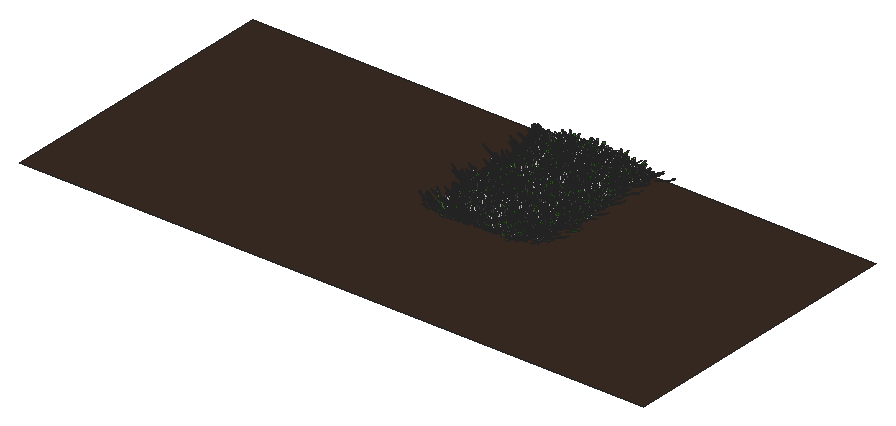
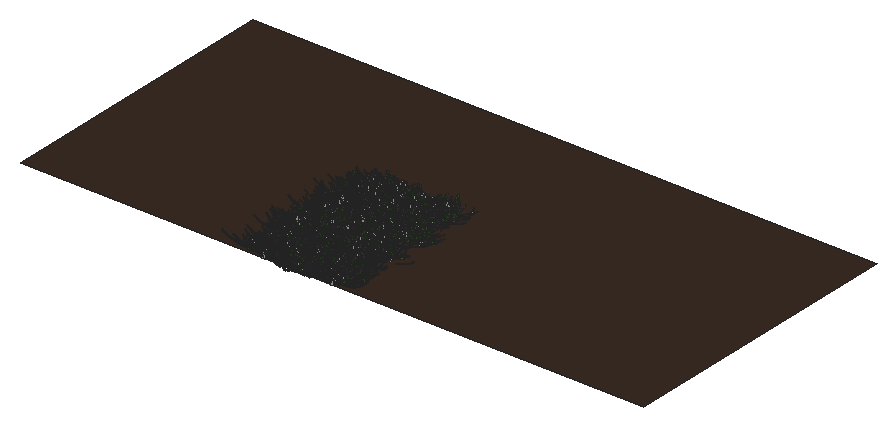
# SketchUp Ruby script. Lengths in inches.
U = 1.inch
M = Sketchup.active_model
def pt(a) = Geom::Point3d.new(a.map { |v| v * U })
def face(e, loops, mat)
  f = e.add_face(loops[0].map { |a| pt(a) })
  loops[1..].each { |l| e.add_face(l.map { |a| pt(a) }).erase! }
  f.material = f.back_material = mat if mat
  f
end
# faces: each face lists its corners as indices into pts; further lists are holes
def faces(e, pts, list, mat = nil) = list.each { |f| face(e, (f[0].is_a?(Array) ? f : [f]).map { |l| l.map { |i| pts[i] } }, mat) }
# xy, xz, yz: faces in a plane at the given z, y or x. An outline is a flat list of corners, or four numbers for a rectangle; further outlines are holes
def ring(l) = l.size == 4 ? [[l[0], l[1]], [l[2], l[1]], [l[2], l[3]], [l[0], l[3]]] : l.each_slice(2).to_a
def flat(e, list, mat, &to3) = list.each { |f| face(e, (f[0].is_a?(Array) ? f : [f]).map { |l| ring(l).map { |u, v| to3.(u, v) } }, mat) }
def xy(e, z, list, mat = nil) = flat(e, list, mat) { |x, y| [x, y, z] }
def xz(e, y, list, mat = nil) = flat(e, list, mat) { |x, z| [x, y, z] }
def yz(e, x, list, mat = nil) = flat(e, list, mat) { |y, z| [x, y, z] }
def lines(e, pts, list) = list.each { |a, b| e.add_line(pt(pts[a]), pt(pts[b])) }
# prism: a flat outline (further loops are holes) pulled along v
def prism(e, loops, v, mat = nil)
  f = face(e, loops, mat); d = Geom::Vector3d.new(v.map { |x| x * U })
  f.pushpull(f.normal.samedirection?(d) ? d.length : -d.length)
end
def box(e, o, s, mat = nil) = prism(e, [[o, [o[0] + s[0], o[1], o[2]], [o[0] + s[0], o[1] + s[1], o[2]], [o[0], o[1] + s[1], o[2]]]], [0, 0, s[2]], mat)
def at(x, y, z, deg = 0) = Geom::Transformation.translation(pt([x, y, z])) * Geom::Transformation.rotation(ORIGIN, Z_AXIS, deg.degrees)
def axes(o, x, y, z) = Geom::Transformation.new([*x, 0, *y, 0, *z, 0, *pt(o).to_a, 1])
def part(name) = M.definitions.add(name)
# library, detail: a bought-in or finely detailed component or shape, given as its bounding box
def library(name, o, s) = part(name).tap { |d| box(d.entities, o, s) }
def detail(e, o, s) = box(e.add_group.entities, o, s)
def put(e, d, t, mat = nil) = e.add_instance(d, t).tap { |i| i.material = mat if mat }
def group(e, t, mat = nil) = e.add_group.tap { |g| g.transformation = t; g.material = mat if mat }.entities
root = M.entities
M.materials.add("Material82").color = [68, 110, 58]
M.materials.add("Material83").color = [48, 90, 38]
M.materials.add("Material84").color = [68, 110, 48]
M.materials.add("Material85").color = [48, 90, 48]
M.materials.add("Material86").color = [58, 110, 58]
M.materials.add("Material87").color = [58, 90, 38]
M.materials.add("Material88").color = [68, 100, 58]
M.materials.add("Material89").color = [48, 100, 38]
M.materials.add("top-soil").color = [58, 44, 36]
c1 = part("grass00")
p = [[-0.6875,0.15,0],[-0.56,0.08,5.52],[-0.04,0.03,2.76],[0.48,-0.02,0],[0.35,-0.02,5.52],[-0.1,-0.14,5.52],
  [-0.12,0.65,8.37],[-0.42,0.65,8.37]]
faces(c1.entities,p,[[0,1,2,3],[3,2,4],[1,5,2],[5,4,2],[1,6,5],[4,5,6],[7,6,1]])
c2 = part("Group16\#1")
put(c2.entities,c1,axes([1.44,-0.61,-0.01],[0.05352,0.12609,0],[-0.10704,0.04543,0.07239],[0.06664,-0.02828,0.11628]),"Material85")
put(c2.entities,c1,axes([0.76,-0.15,-0.01],[0.04676,0.24062,0],[-0.23162,0.04501,0.06642],[0.0652,-0.01267,0.23595]),"Material82")
put(c2.entities,c1,axes([0.79,0.01,-0.01],[-0.00606,0.34651,0],[-0.34381,-0.00602,0.0432],[0.04319,0.00076,0.34386]))
put(c2.entities,c1,axes([1,0.23,-0.01],[-0.07192,0.31144,0],[-0.28722,-0.06632,0.1236],[0.12043,0.02781,0.29478]),"Material84")
put(c2.entities,c1,axes([1.66,0.77,-0.01],[-0.13828,0.29651,0],[-0.21551,-0.1005,0.22471],[0.20365,0.09498,0.23779]),"Material89")
put(c2.entities,c1,axes([0.6875,0.52,-0.01],[-0.18126,0.24051,0],[-0.22746,-0.17142,0.09788],[0.07817,0.05891,0.28481]),"Material84")
put(c2.entities,c1,axes([0.68,0.78,-0.01],[-0.215,0.18688,0],[-0.12385,-0.14248,0.21334],[0.13995,0.16101,0.18878]),"Material82")
put(c2.entities,c1,axes([0.56,1,-0.01],[-0.13756,0.07624,0],[-0.06159,-0.11112,0.0927],[0.04494,0.08108,0.12705]),"Material84")
put(c2.entities,c1,axes([0.2,0.64,-0.01],[-0.23729,0.07254,0],[-0.05711,-0.18681,0.153],[0.04473,0.14632,0.19535]),"Material89")
put(c2.entities,c1,axes([0.0625,0.72,-0.01],[-0.28874,0.02525,0],[-0.02179,-0.24916,0.14647],[0.01276,0.14591,0.25012]),"Material82")
put(c2.entities,c1,axes([-0.08,0.62,-0.01],[-0.34089,-0.04187,0],[0.03255,-0.26504,0.216],[-0.02633,0.21439,0.26703]),"Material89")
put(c2.entities,c1,axes([-0.34,0.98,-0.01],[-0.14314,-0.0493,0],[0.04397,-0.12769,0.06843],[-0.02228,0.0647,0.13505]),"Material89")
put(c2.entities,c1,axes([-0.87,1.45,-0.01],[-0.23488,-0.14114,0],[0.13761,-0.22901,0.06087],[-0.03135,0.05217,0.26717]))
put(c2.entities,c1,axes([-0.72,0.77,-0.01],[-0.14208,-0.13251,0],[0.07209,-0.0773,0.16301],[-0.11118,0.11922,0.1057]),"Material89")
put(c2.entities,c1,axes([-0.62,0.43,-0.01],[-0.14845,-0.21203,0],[0.18654,-0.13061,0.12304],[-0.10079,0.07057,0.22772]),"Material82")
put(c2.entities,c1,axes([-0.68,0.29,-0.01],[-0.13639,-0.32136,0],[0.31723,-0.13464,0.05579],[-0.05136,0.0218,0.34462]),"Material83")
put(c2.entities,c1,axes([-0.64,0.125,-0.01],[-0.0458,-0.23569,0],[0.22124,-0.043,0.08276],[-0.08124,0.01579,0.22538]),"Material86")
put(c2.entities,c1,axes([-1.6,-0.03,-0.01],[0.00576,-0.32897,0],[0.27526,0.00482,0.18018],[-0.18015,-0.00315,0.2753]),"Material84")
put(c2.entities,c1,axes([-1.36,-0.31,-0.01],[0.05718,-0.24765,0],[0.18172,0.04196,0.17267],[-0.16825,-0.03885,0.1865]),"Material89")
put(c2.entities,c1,axes([-1.54,-0.72,-0.01],[0.06537,-0.14017,0],[0.13555,0.06321,0.03939],[-0.0357,-0.01665,0.14956]))
put(c2.entities,c1,axes([-1.19,-0.9,-0.01],[0.09597,-0.12735,0],[0.11214,0.08451,0.07557],[-0.06035,-0.04548,0.14042]),"Material88")
put(c2.entities,c1,axes([-0.47,-0.54,-0.01],[0.11588,-0.10072,0],[0.0618,0.0711,0.12124],[-0.07953,-0.0915,0.0942]))
put(c2.entities,c1,axes([-0.47,-0.84,-0.01],[0.11927,-0.0661,0],[0.06603,0.11913,0.00646],[-0.00313,-0.00565,0.13621]),"Material84")
put(c2.entities,c1,axes([-0.38,-1.24,-0.01],[0.28037,-0.08571,0],[0.0618,0.20215,0.20315],[-0.05939,-0.19428,0.21139]),"Material88")
put(c2.entities,c1,axes([-0.06,-0.66,-0.01],[0.22719,-0.01987,0],[0.01247,0.14255,0.17758],[-0.01547,-0.17691,0.1431]),"Material87")
put(c2.entities,c1,axes([0.11,-0.89,-0.01],[0.14882,0.01828,0],[-0.01058,0.08611,0.12229],[0.01491,-0.12138,0.08676]),"Material85")
put(c2.entities,c1,axes([0.25,-0.72,-0.01],[0.20481,0.07053,0],[-0.06206,0.18022,0.10291],[0.03351,-0.0973,0.1906]),"Material85")
put(c2.entities,c1,axes([0.85,-1.42,-0.01],[0.16481,0.09904,0],[-0.09472,0.15762,0.05616],[0.02893,-0.04814,0.18389]),"Material84")
put(c2.entities,c1,axes([1.01,-1.09,-0.01],[0.21858,0.20385,0],[-0.17495,0.1876,0.15339],[0.10462,-0.11218,0.25652]),"Material89")
put(c2.entities,c1,axes([1.01,-0.71,-0.01],[0.08733,0.12473,0],[-0.06445,0.04512,0.13037],[0.1068,-0.07477,0.07867]),"Material85")
c3 = part("Group15\#1")
put(c3.entities,c2,at(0,0,0))
c4 = part("3darcstudiotree_grass00\#1")
put(c4.entities,c3,at(0,0,0))
xy(root,-29.74,[[596.27,940.12,839.3,1053.55]],"top-soil")
put(root,c4,axes([716.37,1016.65,-29.74],[4.10776,0.45174,0],[-0.96091,1.35899,-0.03867],[-0.06802,0.0962,1.75619]))
put(root,c4,axes([716.7,1044.86,-29.74],[0.30119,1.56993,0],[-3.74927,0.11187,-0.04286],[-0.21599,0.00644,1.42447]))
put(root,c4,axes([718.33,1014.64,-29.74],[-3.02492,-1.16677,0],[2.80082,-1.12934,-0.0483],[0.17838,-0.07192,1.58573]))
put(root,c4,axes([717.53,1046.92,-29.74],[3.50639,-1.07574,0],[2.8139,1.42651,-0.05588],[0.16686,0.08459,1.67045]))
put(root,c4,axes([717.03,996.91,-29.74],[-0.3994,1.69229,0],[-4.36532,-0.16024,-0.02425],[-0.12976,-0.00476,1.76617]))
put(root,c4,axes([718.91,1050.84,-29.74],[-0.91614,-1.55858,0],[4.47177,-0.40881,-0.01344],[0.0544,-0.00497,1.42931]))
put(root,c4,axes([718.23,1031.09,-29.74],[-3.80907,0.85988,0],[-1.7501,-1.20575,-0.03218],[-0.10036,-0.06914,1.65786]))
put(root,c4,axes([718.77,1001.97,-29.74],[1.67083,-1.60234,0],[3.7829,0.6135,-0.00107],[0.00454,0.00074,1.41133]))
put(root,c4,axes([718.07,1049.21,-29.74],[-1.98309,1.36521,0],[-3.29696,-0.74485,-0.00674],[-0.03007,-0.00679,1.46389]))
put(root,c4,axes([718.36,1011.9,-29.74],[-1.6341,1.38385,0],[-3.29524,-0.60518,-0.01596],[-0.09907,-0.01819,1.86544]))
put(root,c4,axes([718.59,1017.96,-29.74],[-1.88391,1.25543,0],[-3.77395,-0.8808,-0.04665],[-0.1806,-0.04215,1.47851]))
put(root,c4,axes([719.67,1041.09,-29.74],[-3.20908,-0.65771,0],[1.52004,-1.1535,-0.02241],[0.0705,-0.0535,1.68548]))
put(root,c4,axes([718.79,1030.31,-29.74],[2.49471,1.02577,0],[-2.71621,1.02741,-0.02632],[-0.13149,0.04974,1.95302]))
put(root,c4,axes([719.14,1037.94,-29.74],[4.09109,-0.59758,0],[1.20224,1.2801,-0.03178],[0.07676,0.08173,1.80429]))
put(root,c4,axes([718.95,1005.53,-29.74],[2.32026,0.93484,0],[-2.86948,1.10768,-0.01876],[-0.07886,0.03044,1.77063]))
put(root,c4,axes([719.68,1024.48,-29.74],[0.18236,1.53314,0],[-4.12116,0.07624,-0.04808],[-0.2649,0.0049,1.70557]))
put(root,c4,axes([719.14,1028.03,-29.74],[1.69594,1.55136,0],[-4.25972,0.72425,-0.01792],[-0.06344,0.01079,1.34035]))
put(root,c4,axes([721.83,1040.77,-29.74],[-0.92548,-1.44714,0],[3.73119,-0.37112,-0.02503],[0.12441,-0.01237,1.47852]))
put(root,c4,axes([721.37,1011.59,-29.74],[-3.65717,1.04753,0],[-2.10189,-1.14131,-0.02785],[-0.11272,-0.06121,1.84622]))
put(root,c4,axes([721.35,1023.08,-29.74],[2.69686,-1.18339,0],[2.47302,0.87653,-0.01288],[0.05957,0.02111,1.54961]))
put(root,c4,axes([722.22,1016.28,-29.74],[-3.84397,-0.38485,0],[1.07963,-1.67717,-0.00944],[0.01366,-0.02122,1.93444]))
put(root,c4,axes([722.0625,1009.79,-29.74],[-1.0379,-1.53247,0],[3.79206,-0.39944,-0.04991],[0.21721,-0.02288,1.32514]))
put(root,c4,axes([722.2,1007.98,-29.74],[1.97874,-1.59829,0],[3.60248,0.69366,-0.03421],[0.19371,0.0373,1.89316]))
put(root,c4,axes([721.41,1025.5625,-29.74],[1.07752,1.49554,0],[-4.17421,0.46775,-0.01918],[-0.10688,0.01198,1.88463]))
put(root,c4,axes([722.91,1038.75,-29.74],[-3.20067,0.8851,0],[-2.09814,-1.18003,-0.04222],[-0.15558,-0.0875,1.75818]))
put(root,c4,axes([723.9,1034.17,-29.74],[-3.27374,-0.87824,0],[2.36689,-1.37221,-0.01911],[0.04526,-0.02624,1.32815]))
put(root,c4,axes([723.5625,1005.6,-29.74],[-0.05891,-1.32731,0],[4.1482,-0.02863,-0.04239],[0.194,-0.00134,1.42343]))
put(root,c4,axes([723.61,1042.43,-29.74],[-3.68407,-0.02356,0],[0.06081,-1.47897,-0.00434],[0.00034,-0.00838,1.37632]))
put(root,c4,axes([722.3,1051.3,-29.74],[3.58378,0.39823,0],[-1.22974,1.72119,-0.04858],[-0.06101,0.08539,1.57379]))
put(root,c4,axes([724.37,1021.25,-29.74],[-0.12973,-1.5282,0],[4.23676,-0.05594,-0.02714],[0.12341,-0.00163,1.44559]))
put(root,c4,axes([723.93,1030.24,-29.74],[-3.75575,0.69708,0],[-1.71963,-1.441,-0.0027],[-0.006,-0.00502,1.57765]))
put(root,c4,axes([723.98,1049.52,-29.74],[-2.752,0.72492,0],[-2.08218,-1.22939,-0.04884],[-0.13401,-0.07912,1.38796]))
put(root,c4,axes([723.99,999.63,-29.74],[2.6038,-1.3441,0],[3.00735,0.90609,-0.00592],[0.02965,0.00893,1.78738]))
put(root,c4,axes([724.84,1000.67,-29.74],[-2.61082,-1.14432,0],[2.90627,-1.03127,-0.02928],[0.10098,-0.03583,1.35967]))
put(root,c4,axes([725.08,1046.52,-29.74],[-3.67064,-0.9709,0],[1.88491,-1.10833,-0.03319],[0.11926,-0.07012,1.63594]))
put(root,c4,axes([723.79,1035.62,-29.74],[-0.84248,1.5623,0],[-4.12413,-0.34589,-0.02719],[-0.15102,-0.01267,1.79436]))
put(root,c4,axes([724.0625,1026.67,-29.74],[-0.14307,1.431,0],[-4.32963,-0.06732,-0.01193],[-0.07261,-0.00113,1.97773]))
put(root,c4,axes([724.9375,1032.0625,-29.74],[-0.69376,1.57067,0],[-3.29157,-0.22612,-0.03897],[-0.27242,-0.01871,1.77692]))
put(root,c4,axes([724.83,1014.9,-29.74],[-0.09674,1.30199,0],[-3.40883,-0.03939,-0.04664],[-0.25839,-0.00299,1.41669]))
put(root,c4,axes([724.41,997.3125,-29.74],[0.99401,1.39114,0],[-3.81883,0.42439,-0.02067],[-0.11338,0.0126,1.69495]))
put(root,c4,axes([724.77,1019.4375,-29.74],[2.79143,1.2628,0],[-2.51561,0.86486,-0.0286],[-0.15611,0.05367,1.81122]))
put(root,c4,axes([725.02,1003.83,-29.74],[-0.55757,1.6642,0],[-4.56304,-0.23777,-0.03274],[-0.13576,-0.00707,1.44297]))
put(root,c4,axes([724.86,1044.85,-29.74],[3.6798,1.00569,0],[-2.52504,1.43694,-0.01195],[-0.02817,0.01603,1.37528]))
put(root,c4,axes([726.92,1034,-29.74],[-4.22095,0.29279,0],[-0.61258,-1.3735,-0.03096],[-0.02808,-0.06297,1.38775]))
put(root,c4,axes([727.11,1018.77,-29.74],[-3.21861,0.39731,0],[-1.33805,-1.68585,-0.0251],[-0.03563,-0.04489,1.59541]))
put(root,c4,axes([727.63,1049.15,-29.74],[-3.05504,-0.78096,0],[2.06441,-1.25601,-0.04254],[0.14556,-0.08856,1.78955]))
put(root,c4,axes([727.14,1031.19,-29.74],[-2.75394,0.84395,0],[-2.86283,-1.45294,-0.03993],[-0.13572,-0.06888,1.9372]))
put(root,c4,axes([728.01,1037.82,-29.74],[-4.11616,0.08361,0],[-0.21641,-1.65704,-0.00589],[-0.00131,-0.01,1.35922]))
put(root,c4,axes([727.16,1005.03,-29.74],[0.77539,1.49335,0],[-4.15697,0.3357,-0.02758],[-0.13791,0.01114,1.62317]))
put(root,c4,axes([728.92,1051.72,-29.74],[0.31357,-1.68647,0],[3.44554,0.09964,-0.00239],[0.01314,0.00038,1.42634]))
put(root,c4,axes([727.43,1020.25,-29.74],[0.83918,1.59477,0],[-3.76377,0.30803,-0.00381],[-0.02098,0.00172,1.62105]))
put(root,c4,axes([729.14,1042.99,-29.74],[-4.10797,-0.04724,0],[0.09871,-1.33508,-0.0193],[0.00442,-0.0598,1.99558]))
put(root,c4,axes([729.1875,1013.81,-29.74],[-4.69627,0.21945,0],[-0.46002,-1.53114,-0.03012],[-0.01578,-0.05252,1.30483]))
put(root,c4,axes([728.11,1001,-29.74],[-1.57534,1.27293,0],[-3.92925,-0.75629,-0.02753],[-0.13899,-0.02675,1.84121]))
put(root,c4,axes([728.49,1003.97,-29.74],[2.05797,-1.09603,0],[2.87826,0.84054,-0.04843],[0.25021,0.07307,1.72564]))
put(root,c4,axes([729.18,1046.3125,-29.74],[0.58086,-1.47611,0],[3.37891,0.2068,-0.00401],[0.02817,0.00172,1.82024]))
put(root,c4,axes([729.51,1023.3,-29.74],[1.23956,-1.20185,0],[3.42028,0.54865,-0.0011],[0.00669,0.00107,1.80895]))
put(root,c4,axes([729.56,1011.9375,-29.74],[0.89327,-1.81074,0],[4.0321,0.30937,-0.02432],[0.12035,0.00923,1.55217]))
put(root,c4,axes([730.45,1009.77,-29.74],[0.20119,-1.37174,0],[3.84475,0.0877,-0.03098],[0.16829,0.00384,1.57088]))
put(root,c4,axes([730.93,1027.92,-29.74],[-3.63168,-0.94551,0],[2.04917,-1.22414,-0.0411],[0.11661,-0.06966,1.43569]))
put(root,c4,axes([730.8,1008.55,-29.74],[-0.37192,-1.4591,0],[3.79295,-0.15037,-0.02999],[0.19954,-0.00791,1.91089]))
put(root,c4,axes([730.53,1024.8,-29.74],[2.01038,-1.40201,0],[3.67214,0.81896,-0.04614],[0.18867,0.04208,1.48544]))
put(root,c4,axes([730.55,998.42,-29.74],[3.21693,-1.31198,0],[2.89205,1.10289,-0.03201],[0.144,0.05492,1.88682]))
put(root,c4,axes([730.1,1041.03,-29.74],[4.09331,0.01199,0],[-0.0289,1.53398,-0.04293],[-0.00148,0.07869,1.35522]))
put(root,c4,axes([730.58,1028.8125,-29.74],[3.51633,-0.36112,0],[0.9428,1.4278,-0.03218],[0.03818,0.05783,1.32043]))
put(root,c4,axes([730.79,1036.08,-29.74],[3.55776,-0.23199,0],[0.75341,1.79699,-0.01648],[0.0118,0.02815,1.51991]))
put(root,c4,axes([730.93,1045.42,-29.74],[-0.04316,1.58062,0],[-4.72981,-0.02009,-0.05791],[-0.26281,-0.00112,1.60897]))
put(root,c4,axes([730.77,1015.79,-29.74],[4.6177,0.37892,0],[-0.96466,1.82835,-0.01168],[-0.00936,0.01774,1.39591]))
put(root,c4,axes([732.97,998.21,-29.74],[2.466,-1.02389,0],[3.09141,1.158,-0.03691],[0.15975,0.05984,1.90749]))
put(root,c4,axes([733.94,1021.22,-29.74],[-2.89327,-0.98526,0],[2.3422,-1.06973,-0.01919],[0.0931,-0.04252,1.99409]))
put(root,c4,axes([732.33,1051.875,-29.74],[4.65922,-0.05932,0],[0.11762,1.43686,-0.01793],[0.0038,0.04639,1.79317]))
put(root,c4,axes([734.1875,1006.3125,-29.74],[-3.01308,-1.39849,0],[3.33443,-1.11734,-0.06095],[0.24941,-0.08358,1.76096]))
put(root,c4,axes([734.03,1043.12,-29.74],[0.00434,-1.45328,0],[3.77222,0.00175,-0.01884],[0.09694,0.00004,1.45492]))
put(root,c4,axes([734.03,1010.48,-29.74],[1.17396,-1.50467,0],[4.45897,0.54108,-0.02541],[0.10297,0.01249,1.48254]))
put(root,c4,axes([734.01,1044.97,-29.74],[-3.66261,0.69653,0],[-1.57298,-1.28643,-0.02015],[-0.06083,-0.04975,1.88684]))
put(root,c4,axes([734.73,1016.42,-29.74],[-3.89542,-0.50736,0],[1.22292,-1.46031,-0.04962],[0.09609,-0.11475,1.8049]))
put(root,c4,axes([734.11,1008.33,-29.74],[-2.84312,0.65512,0],[-2.18872,-1.47733,-0.05376],[-0.11522,-0.07777,1.38154]))
put(root,c4,axes([733.61,1019.12,-29.74],[-0.91872,1.71096,0],[-4.38194,-0.36595,-0.05285],[-0.26515,-0.02214,1.72177]))
put(root,c4,axes([735.08,1053.02,-29.74],[-1.59587,-1.14266,0],[4.12201,-0.89537,-0.06742],[0.26463,-0.05748,1.58058]))
put(root,c4,axes([734.37,1027.27,-29.74],[-2.79487,1.34009,0],[-3.4856,-1.13062,-0.01702],[-0.07434,-0.02411,1.91367]))
put(root,c4,axes([734.16,1048.65,-29.74],[4.14299,-0.56741,0],[1.47163,1.6712,-0.03586],[0.0631,0.07166,1.80381]))
put(root,c4,axes([734.34,1001.45,-29.74],[4.14821,-0.06928,0],[0.17152,1.59736,-0.02002],[0.00473,0.044,1.69539]))
put(root,c4,axes([735.65,1038.57,-29.74],[-4.14933,0.35699,0],[-0.86081,-1.55612,-0.03649],[-0.04634,-0.08377,1.80375]))
put(root,c4,axes([734.32,1033.55,-29.74],[4.28763,0.74332,0],[-1.60811,1.44267,-0.02572],[-0.05083,0.0456,1.47108]))
put(root,c4,axes([736.2,1013.68,-29.74],[-3.82686,-0.23596,0],[0.71117,-1.79387,-0.04342],[0.03245,-0.08186,1.66984]))
put(root,c4,axes([735.125,1024.92,-29.74],[-1.95951,1.68141,0],[-3.84767,-0.6974,-0.02861],[-0.15441,-0.02799,1.88512]))
put(root,c4,axes([736.04,1030.23,-29.74],[-0.85342,-1.31702,0],[3.52172,-0.35493,-0.03508],[0.23842,-0.02403,1.91126]))
put(root,c4,axes([736.25,1011.45,-29.74],[-3.45153,-0.0864,0],[0.28769,-1.78743,-0.04372],[0.01068,-0.06634,1.31241]))
put(root,c4,axes([735.83,1032.29,-29.74],[-1.89755,1.14164,0],[-2.79539,-0.72263,-0.04],[-0.1948,-0.05036,1.45882]))
put(root,c4,axes([736.39,1040.67,-29.74],[-4.56188,0.50767,0],[-1.2186,-1.7031,-0.00145],[-0.00214,-0.00299,1.8291]))
put(root,c4,axes([735.27,1047.56,-29.74],[-0.0946,1.80399,0],[-4.6355,-0.03781,-0.04199],[-0.20347,-0.00166,1.68448]))
put(root,c4,axes([735.53,1035.81,-29.74],[3.68176,-0.08889,0],[0.28452,1.83295,-0.0507],[0.01477,0.09515,1.66388]))
put(root,c4,axes([735.65,1022.99,-29.74],[1.28845,1.74913,0],[-3.19455,0.36599,-0.00931],[-0.04886,0.0056,1.3628]))
put(root,c4,axes([736.41,1004.1,-29.74],[3.2366,-0.57131,0],[1.58048,1.39258,-0.04939],[0.12568,0.11074,1.80606]))
put(root,c4,axes([738.06,1032.03,-29.74],[-3.02696,1.26281,0],[-2.89442,-1.07905,-0.01805],[-0.07526,-0.02806,1.71251]))
put(root,c4,axes([738.51,1025.5,-29.74],[-3.18632,0.63668,0],[-1.6075,-1.25121,-0.00642],[-0.0144,-0.01121,1.3229]))
put(root,c4,axes([739.14,1001.04,-29.74],[-3.56938,-0.43544,0],[1.36231,-1.73682,-0.06046],[0.07694,-0.09809,1.48798]))
put(root,c4,axes([738.36,1035.32,-29.74],[-2.26269,0.97698,0],[-3.46591,-1.24844,-0.00484],[-0.01583,-0.0057,1.55938]))
put(root,c4,axes([738.68,998.84,-29.74],[-3.08205,1.07293,0],[-3.11637,-1.39229,-0.01862],[-0.0666,-0.02976,1.90809]))
put(root,c4,axes([739.86,1029.41,-29.74],[-1.06768,-1.28552,0],[4.42505,-0.5716,-0.01545],[0.0652,-0.00842,1.54954]))
put(root,c4,axes([739.92,997.44,-29.74],[-0.50603,-1.39331,0],[4.58553,-0.25902,-0.00214],[0.00976,-0.00055,1.59988]))
put(root,c4,axes([738.65,1016.83,-29.74],[-2.17882,1.11223,0],[-3.27984,-0.99929,-0.01374],[-0.05934,-0.01808,1.69563]))
put(root,c4,axes([738.3125,1005.88,-29.74],[-1.12838,1.66356,0],[-4.06225,-0.42855,-0.00132],[-0.00752,-0.00079,1.858]))
put(root,c4,axes([737.92,1023.17,-29.74],[3.24771,1.22669,0],[-3.17033,1.30544,-0.01961],[-0.06543,0.02694,1.65716]))
put(root,c4,axes([739.77,1003.25,-29.74],[-3.65901,0.17551,0],[-0.56536,-1.83311,-0.00408],[-0.00246,-0.00797,1.74968]))
put(root,c4,axes([738.35,1045.58,-29.74],[0.64791,1.78613,0],[-4.32576,0.24405,-0.02596],[-0.10407,0.00587,1.32635]))
put(root,c4,axes([738.57,1026.68,-29.74],[-1.07809,1.72568,0],[-4.31745,-0.4195,-0.00818],[-0.04348,-0.00422,1.82396]))
put(root,c4,axes([738.875,1047.25,-29.74],[2.43664,1.45627,0],[-2.82206,0.73439,-0.04277],[-0.22349,0.05816,1.58679]))
put(root,c4,axes([739.53,1038.88,-29.74],[4.1241,0.10126,0],[-0.23149,1.46627,-0.04181],[-0.01816,0.11501,1.95138]))
put(root,c4,axes([740.76,1050.66,-29.74],[-3.5428,1.01388,0],[-2.21614,-1.2044,-0.01293],[-0.05166,-0.02807,1.92389]))
put(root,c4,axes([739.5,1020.17,-29.74],[2.96136,1.19987,0],[-3.11013,1.19384,-0.004],[-0.01667,0.0064,1.89371]))
put(root,c4,axes([741.3,1010.4375,-29.74],[-4.14748,0.25836,0],[-0.59761,-1.49206,-0.01239],[-0.00958,-0.02393,1.42361]))
put(root,c4,axes([740.05,1007.84,-29.74],[4.21182,0.14848,0],[-0.32581,1.4374,-0.01038],[-0.00654,0.02884,1.94021]))
put(root,c4,axes([740.06,1033.9,-29.74],[4.10391,0.70985,0],[-1.57565,1.41679,-0.04488],[-0.12117,0.10895,1.97665]))
put(root,c4,axes([740.18,1012.47,-29.74],[1.10995,1.51966,0],[-3.58981,0.40779,-0.02733],[-0.15418,0.01751,1.64375]))
put(root,c4,axes([741.21,1048.79,-29.74],[2.20641,-0.98098,0],[3.35125,1.17232,-0.037],[0.12603,0.04409,1.52862]))
put(root,c4,axes([741.11,1042.75,-29.74],[2.40726,1.00896,0],[-2.45133,0.90962,-0.04643],[-0.23456,0.08704,1.7498]))
put(root,c4,axes([741.1,1040.88,-29.74],[1.86032,1.34861,0],[-2.96544,0.63621,-0.01685],[-0.11323,0.02429,1.93576]))
put(root,c4,axes([741.36,1019.48,-29.74],[4.19014,0.72772,0],[-1.46084,1.30821,-0.04159],[-0.08773,0.07856,1.42181]))
put(root,c4,axes([743.4,1007.11,-29.74],[-1.84068,-1.59832,0],[3.91902,-0.70195,-0.02239],[0.11993,-0.02148,1.89813]))
put(root,c4,axes([741.93,1013.75,-29.74],[0.99879,1.74855,0],[-3.87665,0.3444,-0.04632],[-0.24296,0.02158,1.6013]))
put(root,c4,axes([743.86,1036.375,-29.74],[-4.27172,-0.34301,0],[0.88739,-1.71879,-0.03896],[0.04123,-0.07985,1.76791]))
put(root,c4,axes([743.55,1034.52,-29.74],[3.05285,-0.84724,0],[2.57962,1.44566,-0.04926],[0.16288,0.09128,1.93034]))
put(root,c4,axes([743.85,1040.04,-29.74],[-2.93173,0.8474,0],[-2.63832,-1.41962,-0.02359],[-0.06961,-0.03745,1.66971]))
put(root,c4,axes([744.91,1050.04,-29.74],[-4.04158,-0.94067,0],[1.75814,-1.17484,-0.01139],[0.03404,-0.02275,1.52439]))
put(root,c4,axes([745.02,1000.93,-29.74],[-0.45548,-1.68091,0],[3.45741,-0.14571,-0.01446],[0.0889,-0.00375,1.61179]))
put(root,c4,axes([744.47,999.58,-29.74],[-3.13157,0.80525,0],[-2.19448,-1.32731,-0.02083],[-0.06068,-0.0367,1.60618]))
put(root,c4,axes([745.37,1046.52,-29.74],[-3.80321,-0.44648,0],[1.10938,-1.46975,-0.0137],[0.0187,-0.02478,1.39479]))
put(root,c4,axes([745.72,1020.97,-29.74],[-3.37995,-1.26993,0],[3.24999,-1.34532,-0.03405],[0.09733,-0.04029,1.46358]))
put(root,c4,axes([743.75,1012.8125,-29.74],[1.40547,1.51439,0],[-4.0139,0.57938,-0.03042],[-0.14333,0.02069,1.60735]))
put(root,c4,axes([744.18,1027.1875,-29.74],[4.00543,0.63259,0],[-1.51384,1.49079,-0.05201],[-0.11143,0.10973,1.75905]))
put(root,c4,axes([745.14,1044.91,-29.74],[3.22644,-0.51746,0],[1.32565,1.28555,-0.02601],[0.05462,0.05297,1.4702]))
put(root,c4,axes([744.9,1038.28,-29.74],[4.21739,-0.2744,0],[0.59088,1.41243,-0.03976],[0.04192,0.1002,1.7619]))
put(root,c4,axes([745.37,1005.62,-29.74],[-0.09951,1.54184,0],[-3.8951,-0.0391,-0.03168],[-0.18001,-0.00181,1.66016]))
put(root,c4,axes([745.9,1023.28,-29.74],[3.13004,-0.71111,0],[2.12935,1.45771,-0.00508],[0.01244,0.00852,1.56982]))
put(root,c4,axes([745.47,1018.96,-29.74],[1.71903,1.73474,0],[-3.69921,0.57012,-0.05423],[-0.23247,0.03583,1.37014]))
put(root,c4,axes([746.89,1014.42,-29.74],[1.52517,-1.72025,0],[3.68343,0.50792,-0.01723],[0.07984,0.01101,1.43549]))
put(root,c4,axes([746.45,1003.85,-29.74],[-2.42659,1.57566,0],[-3.75552,-0.89953,-0.06137],[-0.23264,-0.05572,1.46064]))
put(root,c4,axes([746.13,1009.48,-29.74],[3.59244,-0.46408,0],[1.16578,1.40355,-0.03684],[0.0661,0.07959,1.61813]))
put(root,c4,axes([746.35,1051.23,-29.74],[4.25801,-0.4781,0],[1.08249,1.49942,-0.0361],[0.05003,0.0693,1.4995]))
put(root,c4,axes([747.28,1015.99,-29.74],[-3.02925,1.34013,0],[-2.7234,-0.95744,-0.02096],[-0.09613,-0.0338,1.6805]))
put(root,c4,axes([747.14,1031.13,-29.74],[-1.53161,1.39817,0],[-3.93212,-0.66992,-0.05011],[-0.24211,-0.04125,1.6899]))
put(root,c4,axes([747.5,1028.89,-29.74],[-2.46131,1.0799,0],[-2.93079,-1.03891,-0.05045],[-0.18868,-0.06689,1.48531]))
